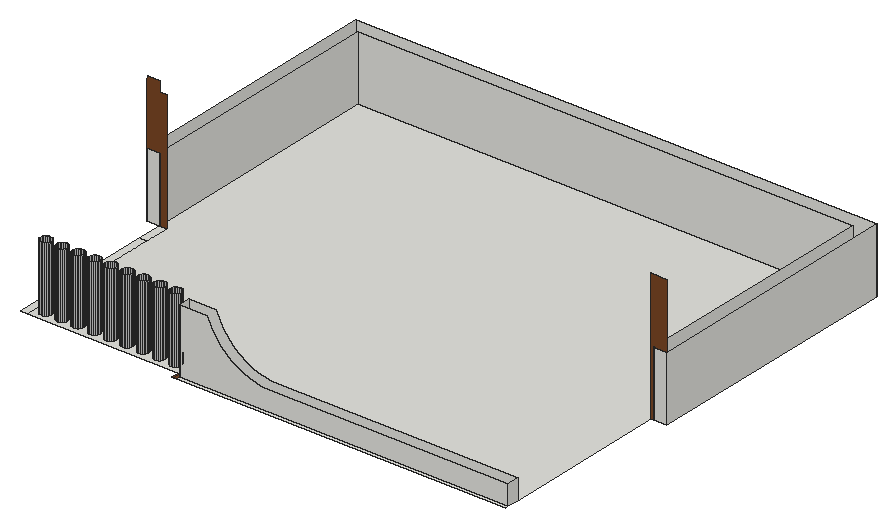
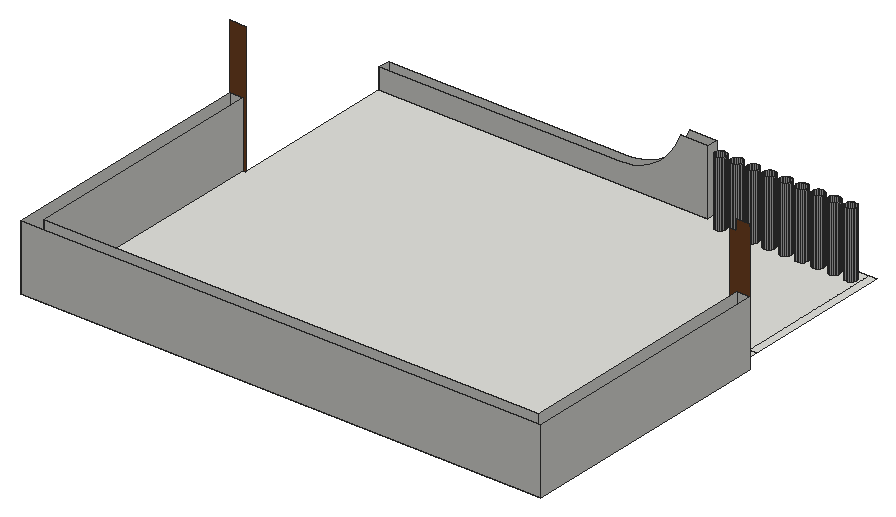
# SketchUp Ruby script. Lengths in millimetres.
U = 1.mm
M = Sketchup.active_model
def pt(a) = Geom::Point3d.new(a.map { |v| v * U })
def face(e, loops, mat)
  f = e.add_face(loops[0].map { |a| pt(a) })
  loops[1..].each { |l| e.add_face(l.map { |a| pt(a) }).erase! }
  f.material = f.back_material = mat if mat
  f
end
# faces: each face lists its corners as indices into pts; further lists are holes
def faces(e, pts, list, mat = nil) = list.each { |f| face(e, (f[0].is_a?(Array) ? f : [f]).map { |l| l.map { |i| pts[i] } }, mat) }
# xy, xz, yz: faces in a plane at the given z, y or x. An outline is a flat list of corners, or four numbers for a rectangle; further outlines are holes
def ring(l) = l.size == 4 ? [[l[0], l[1]], [l[2], l[1]], [l[2], l[3]], [l[0], l[3]]] : l.each_slice(2).to_a
def flat(e, list, mat, &to3) = list.each { |f| face(e, (f[0].is_a?(Array) ? f : [f]).map { |l| ring(l).map { |u, v| to3.(u, v) } }, mat) }
def xy(e, z, list, mat = nil) = flat(e, list, mat) { |x, y| [x, y, z] }
def xz(e, y, list, mat = nil) = flat(e, list, mat) { |x, z| [x, y, z] }
def yz(e, x, list, mat = nil) = flat(e, list, mat) { |y, z| [x, y, z] }
def lines(e, pts, list) = list.each { |a, b| e.add_line(pt(pts[a]), pt(pts[b])) }
# prism: a flat outline (further loops are holes) pulled along v
def prism(e, loops, v, mat = nil)
  f = face(e, loops, mat); d = Geom::Vector3d.new(v.map { |x| x * U })
  f.pushpull(f.normal.samedirection?(d) ? d.length : -d.length)
end
def box(e, o, s, mat = nil) = prism(e, [[o, [o[0] + s[0], o[1], o[2]], [o[0] + s[0], o[1] + s[1], o[2]], [o[0], o[1] + s[1], o[2]]]], [0, 0, s[2]], mat)
def at(x, y, z, deg = 0) = Geom::Transformation.translation(pt([x, y, z])) * Geom::Transformation.rotation(ORIGIN, Z_AXIS, deg.degrees)
def axes(o, x, y, z) = Geom::Transformation.new([*x, 0, *y, 0, *z, 0, *pt(o).to_a, 1])
def part(name) = M.definitions.add(name)
# library, detail: a bought-in or finely detailed component or shape, given as its bounding box
def library(name, o, s) = part(name).tap { |d| box(d.entities, o, s) }
def detail(e, o, s) = box(e.add_group.entities, o, s)
def put(e, d, t, mat = nil) = e.add_instance(d, t).tap { |i| i.material = mat if mat }
def group(e, t, mat = nil) = e.add_group.tap { |g| g.transformation = t; g.material = mat if mat }.entities
root = M.entities
M.materials.add("[Metal Corrugated Shiny]").color = [193, 193, 193]
M.materials.add("[Wood Veneer 01]").color = [120, 70, 37]
xy(root,7289.8,[[[4112.5,514.4,11814.3,514.4,11814.3,582.5,4124.5,582.5,4124.5,849.3,11814.3,849.3,11814.3,4760.9,11890.5,4760.9,11890.5,10572.8,308.1,10572.8,308.1,4760.9,479.5,4760.9,479.5,687.4,4112.5,687.4],[1458.7,818.4,1424.6,822.5,1392.7,835.4,1365.2,856,1344,883.1,1330.5,914.8,1325.6,948.8,1329.8,983,1342.6,1014.9,1363.3,1042.4,1390.3,1063.6,1422,1077.1,1456,1081.9,1490.2,1077.8,1522.1,1064.9,1549.6,1044.3,1570.8,1017.2,1584.3,985.6,1589.1,951.5,1585,917.4,1572.2,885.5,1551.5,858,1524.4,836.7,1492.8,823.2],[1839.7,818.4,1805.6,822.5,1773.7,835.4,1746.2,856,1725,883.1,1711.5,914.8,1706.6,948.8,1710.8,983,1723.6,1014.9,1744.3,1042.4,1771.3,1063.6,1803,1077.1,1837,1081.9,1871.2,1077.8,1903.1,1064.9,1930.6,1044.3,1951.8,1017.2,1965.3,985.6,1970.1,951.5,1966,917.4,1953.2,885.5,1932.5,858,1905.4,836.7,1873.8,823.2],[2220.7,818.4,2186.6,822.5,2154.7,835.4,2127.2,856,2106,883.1,2092.5,914.8,2087.6,948.8,2091.8,983,2104.6,1014.9,2125.3,1042.4,2152.3,1063.6,2184,1077.1,2218,1081.9,2252.2,1077.8,2284.1,1064.9,2311.6,1044.3,2332.8,1017.2,2346.3,985.6,2351.1,951.5,2347,917.4,2334.2,885.5,2313.5,858,2286.4,836.7,2254.8,823.2],[1077.7,818.4,1043.6,822.5,1011.7,835.4,984.2,856,963,883.1,949.5,914.8,944.6,948.8,948.8,983,961.6,1014.9,982.3,1042.4,1009.3,1063.6,1041,1077.1,1075,1081.9,1109.2,1077.8,1141.1,1064.9,1168.6,1044.3,1189.8,1017.2,1203.3,985.6,1208.1,951.5,1204,917.4,1191.2,885.5,1170.5,858,1143.4,836.7,1111.8,823.2],[696.7,818.4,662.6,822.5,630.7,835.4,603.2,856,582,883.1,568.5,914.8,563.6,948.8,567.8,983,580.6,1014.9,601.3,1042.4,628.3,1063.6,660,1077.1,694,1081.9,728.2,1077.8,760.1,1064.9,787.6,1044.3,808.8,1017.2,822.3,985.6,827.1,951.5,823,917.4,810.2,885.5,789.5,858,762.4,836.7,730.8,823.2],[2601.7,818.4,2567.6,822.5,2535.7,835.4,2508.2,856,2487,883.1,2473.5,914.8,2468.6,948.8,2472.8,983,2485.6,1014.9,2506.3,1042.4,2533.3,1063.6,2565,1077.1,2599,1081.9,2633.2,1077.8,2665.1,1064.9,2692.6,1044.3,2713.8,1017.2,2727.3,985.6,2732.1,951.5,2728,917.4,2715.2,885.5,2694.5,858,2667.4,836.7,2635.8,823.2],[2982.7,818.4,2948.6,822.5,2916.7,835.4,2889.2,856,2868,883.1,2854.5,914.8,2849.6,948.8,2853.8,983,2866.6,1014.9,2887.3,1042.4,2914.3,1063.6,2946,1077.1,2980,1081.9,3014.2,1077.8,3046.1,1064.9,3073.6,1044.3,3094.8,1017.2,3108.3,985.6,3113.1,951.5,3109,917.4,3096.2,885.5,3075.5,858,3048.4,836.7,3016.8,823.2],[3363.7,818.4,3329.6,822.5,3297.7,835.4,3270.2,856,3249,883.1,3235.5,914.8,3230.6,948.8,3234.8,983,3247.6,1014.9,3268.3,1042.4,3295.3,1063.6,3327,1077.1,3361,1081.9,3395.2,1077.8,3427.1,1064.9,3454.6,1044.3,3475.8,1017.2,3489.3,985.6,3494.1,951.5,3490,917.4,3477.2,885.5,3456.5,858,3429.4,836.7,3397.8,823.2],[3744.7,818.4,3710.6,822.5,3678.7,835.4,3651.2,856,3630,883.1,3616.5,914.8,3611.6,948.8,3615.8,983,3628.6,1014.9,3649.3,1042.4,3676.3,1063.6,3708,1077.1,3742,1081.9,3776.2,1077.8,3808.1,1064.9,3835.6,1044.3,3856.8,1017.2,3870.3,985.6,3875.1,951.5,3871,917.4,3858.2,885.5,3837.5,858,3810.4,836.7,3778.8,823.2]],[4124.5,582.5,11814.3,849.3],[308.1,687.4,479.5,4181.5],[308.1,4181.5,479.5,4760.9],[3.3,4760.9,3.3,10877.6,12195.3,10877.6,12195.3,4760.9,11890.5,4760.9,11890.5,10572.8,308.1,10572.8,308.1,4760.9]])
xy(root,7289.8,[[696.7,818.4,662.6,822.5,630.7,835.4,603.2,856,582,883.1,568.5,914.8,563.6,948.8,567.8,983,580.6,1014.9,601.3,1042.4,628.3,1063.6,660,1077.1,694,1081.9,728.2,1077.8,760.1,1064.9,787.6,1044.3,808.8,1017.2,822.3,985.6,827.1,951.5,823,917.4,810.2,885.5,789.5,858,762.4,836.7,730.8,823.2],[1077.7,818.4,1043.6,822.5,1011.7,835.4,984.2,856,963,883.1,949.5,914.8,944.6,948.8,948.8,983,961.6,1014.9,982.3,1042.4,1009.3,1063.6,1041,1077.1,1075,1081.9,1109.2,1077.8,1141.1,1064.9,1168.6,1044.3,1189.8,1017.2,1203.3,985.6,1208.1,951.5,1204,917.4,1191.2,885.5,1170.5,858,1143.4,836.7,1111.8,823.2],[1458.7,818.4,1424.6,822.5,1392.7,835.4,1365.2,856,1344,883.1,1330.5,914.8,1325.6,948.8,1329.8,983,1342.6,1014.9,1363.3,1042.4,1390.3,1063.6,1422,1077.1,1456,1081.9,1490.2,1077.8,1522.1,1064.9,1549.6,1044.3,1570.8,1017.2,1584.3,985.6,1589.1,951.5,1585,917.4,1572.2,885.5,1551.5,858,1524.4,836.7,1492.8,823.2],[1839.7,818.4,1805.6,822.5,1773.7,835.4,1746.2,856,1725,883.1,1711.5,914.8,1706.6,948.8,1710.8,983,1723.6,1014.9,1744.3,1042.4,1771.3,1063.6,1803,1077.1,1837,1081.9,1871.2,1077.8,1903.1,1064.9,1930.6,1044.3,1951.8,1017.2,1965.3,985.6,1970.1,951.5,1966,917.4,1953.2,885.5,1932.5,858,1905.4,836.7,1873.8,823.2],[2220.7,818.4,2186.6,822.5,2154.7,835.4,2127.2,856,2106,883.1,2092.5,914.8,2087.6,948.8,2091.8,983,2104.6,1014.9,2125.3,1042.4,2152.3,1063.6,2184,1077.1,2218,1081.9,2252.2,1077.8,2284.1,1064.9,2311.6,1044.3,2332.8,1017.2,2346.3,985.6,2351.1,951.5,2347,917.4,2334.2,885.5,2313.5,858,2286.4,836.7,2254.8,823.2],
  [2601.7,818.4,2567.6,822.5,2535.7,835.4,2508.2,856,2487,883.1,2473.5,914.8,2468.6,948.8,2472.8,983,2485.6,1014.9,2506.3,1042.4,2533.3,1063.6,2565,1077.1,2599,1081.9,2633.2,1077.8,2665.1,1064.9,2692.6,1044.3,2713.8,1017.2,2727.3,985.6,2732.1,951.5,2728,917.4,2715.2,885.5,2694.5,858,2667.4,836.7,2635.8,823.2],[2982.7,818.4,2948.6,822.5,2916.7,835.4,2889.2,856,2868,883.1,2854.5,914.8,2849.6,948.8,2853.8,983,2866.6,1014.9,2887.3,1042.4,2914.3,1063.6,2946,1077.1,2980,1081.9,3014.2,1077.8,3046.1,1064.9,3073.6,1044.3,3094.8,1017.2,3108.3,985.6,3113.1,951.5,3109,917.4,3096.2,885.5,3075.5,858,3048.4,836.7,3016.8,823.2],[3363.7,818.4,3329.6,822.5,3297.7,835.4,3270.2,856,3249,883.1,3235.5,914.8,3230.6,948.8,3234.8,983,3247.6,1014.9,3268.3,1042.4,3295.3,1063.6,3327,1077.1,3361,1081.9,3395.2,1077.8,3427.1,1064.9,3454.6,1044.3,3475.8,1017.2,3489.3,985.6,3494.1,951.5,3490,917.4,3477.2,885.5,3456.5,858,3429.4,836.7,3397.8,823.2],[3744.7,818.4,3710.6,822.5,3678.7,835.4,3651.2,856,3630,883.1,3616.5,914.8,3611.6,948.8,3615.8,983,3628.6,1014.9,3649.3,1042.4,3676.3,1063.6,3708,1077.1,3742,1081.9,3776.2,1077.8,3808.1,1064.9,3835.6,1044.3,3856.8,1017.2,3870.3,985.6,3875.1,951.5,3871,917.4,3858.2,885.5,3837.5,858,3810.4,836.7,3778.8,823.2]],"[Metal Corrugated Shiny]")
xz(root,582.5,[[4124.5,7289.8,11814.3,7289.8,11814.3,7765.4,6213.6,7765.4,6054.6,7773.7,5897.3,7798.5,5743.5,7839.6,5594.8,7896.5,5452.9,7968.5,5319.2,8055,5195.3,8154.9,5082.4,8267.2,4981.9,8390.6,4894.7,8523.8,4822,8665.4,4764.3,8813.8,4124.5,8813.8]])
xz(root,849.3,[[4124.5,7289.8,4124.5,8813.8,4764.3,8813.8,4822,8665.4,4894.7,8523.8,4981.9,8390.6,5082.4,8267.2,5195.3,8154.9,5319.2,8055,5452.9,7968.5,5594.8,7896.5,5743.5,7839.6,5897.3,7798.5,6054.6,7773.7,6213.6,7765.4,11814.3,7765.4,11814.3,7289.8]])
xz(root,4760.9,[[3.3,7289.8,308.1,8813.8],[11890.5,7289.8,12195.3,8813.8]])
xz(root,4760.9,[[308.1,7289.8,308.1,8813.8,3.3,8813.8,3.3,10221.2,7.1,10258.4,24.3,10325.9,29.4,10337.8,308.1,10337.8,308.1,10096.5,479.5,10096.5,479.5,7289.8],[11814.3,7289.8,11814.3,10337.8,12195.3,10337.8,12195.3,8813.8,11890.5,8813.8,11890.5,7289.8]],"[Wood Veneer 01]")
xz(root,10572.8,[[308.1,7289.8,11890.5,8813.8]])
xz(root,10877.6,[[3.3,7289.8,12195.3,8813.8]])
yz(root,3.3,[[4760.9,7289.8,10877.6,8813.8]])
yz(root,308.1,[[4760.9,7289.8,10572.8,8813.8]])
yz(root,4124.5,[[582.5,7289.8,849.3,8813.8]])
yz(root,11814.3,[[582.5,7289.8,849.3,7765.4]])
yz(root,11890.5,[[4760.9,7289.8,10572.8,8813.8]])
yz(root,12195.3,[[4760.9,7289.8,10877.6,8813.8]])
p = [[4048.9,687.4,7286.3],[3986.1,687.4,7276],[3986.1,514.4,7276],[4048.9,514.4,7286.3],[4112.5,687.4,7289.8],[4112.5,514.4,7289.8],
  [662.6,822.5,7289.8],[696.7,818.4,7289.8],[696.7,818.4,8813.8],[662.6,822.5,8813.8],[730.8,823.2,7289.8],[730.8,823.2,8813.8],
  [1043.6,822.5,7289.8],[1077.7,818.4,7289.8],[1077.7,818.4,8813.8],[1043.6,822.5,8813.8],[1111.8,823.2,7289.8],[1111.8,823.2,8813.8],
  [1424.6,822.5,7289.8],[1458.7,818.4,7289.8],[1458.7,818.4,8813.8],[1424.6,822.5,8813.8],[1492.8,823.2,7289.8],[1492.8,823.2,8813.8],
  [1805.6,822.5,7289.8],[1839.7,818.4,7289.8],[1839.7,818.4,8813.8],[1805.6,822.5,8813.8],[1873.8,823.2,7289.8],[1873.8,823.2,8813.8],
  [2186.6,822.5,7289.8],[2220.7,818.4,7289.8],[2220.7,818.4,8813.8],[2186.6,822.5,8813.8],[2254.8,823.2,7289.8],[2254.8,823.2,8813.8],
  [2567.6,822.5,7289.8],[2601.7,818.4,7289.8],[2601.7,818.4,8813.8],[2567.6,822.5,8813.8],[2635.8,823.2,7289.8],[2635.8,823.2,8813.8],
  [2948.6,822.5,7289.8],[2982.7,818.4,7289.8],[2982.7,818.4,8813.8],[2948.6,822.5,8813.8],[3016.8,823.2,7289.8],[3016.8,823.2,8813.8],
  [3329.6,822.5,7289.8],[3363.7,818.4,7289.8],[3363.7,818.4,8813.8],[3329.6,822.5,8813.8],[3397.8,823.2,7289.8],[3397.8,823.2,8813.8],
  [3710.6,822.5,7289.8],[3744.7,818.4,7289.8],[3744.7,818.4,8813.8],[3710.6,822.5,8813.8],[3778.8,823.2,7289.8],[3778.8,823.2,8813.8],
  [630.7,835.4,7289.8],[630.7,835.4,8813.8],[1011.7,835.4,7289.8],[1011.7,835.4,8813.8],[1392.7,835.4,7289.8],[1392.7,835.4,8813.8],
  [1773.7,835.4,7289.8],[1773.7,835.4,8813.8],[2154.7,835.4,7289.8],[2154.7,835.4,8813.8],[2535.7,835.4,7289.8],[2535.7,835.4,8813.8],
  [2916.7,835.4,7289.8],[2916.7,835.4,8813.8],[3297.7,835.4,7289.8],[3297.7,835.4,8813.8],[3678.7,835.4,7289.8],[3678.7,835.4,8813.8],
  [762.4,836.7,7289.8],[762.4,836.7,8813.8],[1143.4,836.7,7289.8],[1143.4,836.7,8813.8],[1524.4,836.7,7289.8],[1524.4,836.7,8813.8],
  [1905.4,836.7,7289.8],[1905.4,836.7,8813.8],[2286.4,836.7,7289.8],[2286.4,836.7,8813.8],[2667.4,836.7,7289.8],[2667.4,836.7,8813.8],
  [3048.4,836.7,7289.8],[3048.4,836.7,8813.8],[3429.4,836.7,7289.8],[3429.4,836.7,8813.8],[3810.4,836.7,7289.8],[3810.4,836.7,8813.8],
  [603.2,856,7289.8],[603.2,856,8813.8],[984.2,856,7289.8],[984.2,856,8813.8],[1365.2,856,7289.8],[1365.2,856,8813.8],
  [1746.2,856,7289.8],[1746.2,856,8813.8],[2127.2,856,7289.8],[2127.2,856,8813.8],[2508.2,856,7289.8],[2508.2,856,8813.8],
  [2889.2,856,7289.8],[2889.2,856,8813.8],[3270.2,856,7289.8],[3270.2,856,8813.8],[3651.2,856,7289.8],[3651.2,856,8813.8],
  [789.5,858,7289.8],[789.5,858,8813.8],[1170.5,858,7289.8],[1170.5,858,8813.8],[1551.5,858,7289.8],[1551.5,858,8813.8],
  [1932.5,858,7289.8],[1932.5,858,8813.8],[2313.5,858,7289.8],[2313.5,858,8813.8],[2694.5,858,7289.8],[2694.5,858,8813.8],
  [3075.5,858,7289.8],[3075.5,858,8813.8],[3456.5,858,7289.8],[3456.5,858,8813.8],[3837.5,858,7289.8],[3837.5,858,8813.8],
  [582,883.1,7289.8],[582,883.1,8813.8],[963,883.1,7289.8],[963,883.1,8813.8],[1344,883.1,7289.8],[1344,883.1,8813.8],
  [1725,883.1,7289.8],[1725,883.1,8813.8],[2106,883.1,7289.8],[2106,883.1,8813.8],[2487,883.1,7289.8],[2487,883.1,8813.8],
  [2868,883.1,7289.8],[2868,883.1,8813.8],[3249,883.1,7289.8],[3249,883.1,8813.8],[3630,883.1,7289.8],[3630,883.1,8813.8],
  [810.2,885.5,7289.8],[810.2,885.5,8813.8],[1191.2,885.5,7289.8],[1191.2,885.5,8813.8],[1572.2,885.5,7289.8],[1572.2,885.5,8813.8],
  [1953.2,885.5,7289.8],[1953.2,885.5,8813.8],[2334.2,885.5,7289.8],[2334.2,885.5,8813.8],[2715.2,885.5,7289.8],[2715.2,885.5,8813.8],
  [3096.2,885.5,7289.8],[3096.2,885.5,8813.8],[3477.2,885.5,7289.8],[3477.2,885.5,8813.8],[3858.2,885.5,7289.8],[3858.2,885.5,8813.8],
  [568.5,914.8,7289.8],[568.5,914.8,8813.8],[949.5,914.8,7289.8],[949.5,914.8,8813.8],[1330.5,914.8,7289.8],[1330.5,914.8,8813.8],
  [1711.5,914.8,7289.8],[1711.5,914.8,8813.8],[2092.5,914.8,7289.8],[2092.5,914.8,8813.8],[2473.5,914.8,7289.8],[2473.5,914.8,8813.8],
  [2854.5,914.8,7289.8],[2854.5,914.8,8813.8],[3235.5,914.8,7289.8],[3235.5,914.8,8813.8],[3616.5,914.8,7289.8],[3616.5,914.8,8813.8],
  [823,917.4,7289.8],[823,917.4,8813.8],[1204,917.4,7289.8],[1204,917.4,8813.8],[1585,917.4,7289.8],[1585,917.4,8813.8],
  [1966,917.4,7289.8],[1966,917.4,8813.8],[2347,917.4,7289.8],[2347,917.4,8813.8],[2728,917.4,7289.8],[2728,917.4,8813.8],
  [3109,917.4,7289.8],[3109,917.4,8813.8],[3490,917.4,7289.8],[3490,917.4,8813.8],[3871,917.4,7289.8],[3871,917.4,8813.8],
  [563.6,948.8,7289.8],[563.6,948.8,8813.8],[944.6,948.8,7289.8],[944.6,948.8,8813.8],[1325.6,948.8,7289.8],[1325.6,948.8,8813.8],
  [1706.6,948.8,7289.8],[1706.6,948.8,8813.8],[2087.6,948.8,7289.8],[2087.6,948.8,8813.8],[2468.6,948.8,7289.8],[2468.6,948.8,8813.8],
  [2849.6,948.8,7289.8],[2849.6,948.8,8813.8],[3230.6,948.8,7289.8],[3230.6,948.8,8813.8],[3611.6,948.8,7289.8],[3611.6,948.8,8813.8],
  [827.1,951.5,7289.8],[827.1,951.5,8813.8],[1208.1,951.5,7289.8],[1208.1,951.5,8813.8],[1589.1,951.5,7289.8],[1589.1,951.5,8813.8],
  [1970.1,951.5,7289.8],[1970.1,951.5,8813.8],[2351.1,951.5,7289.8],[2351.1,951.5,8813.8],[2732.1,951.5,7289.8],[2732.1,951.5,8813.8],
  [3113.1,951.5,7289.8],[3113.1,951.5,8813.8],[3494.1,951.5,7289.8],[3494.1,951.5,8813.8],[3875.1,951.5,7289.8],[3875.1,951.5,8813.8],
  [567.8,983,7289.8],[567.8,983,8813.8],[948.8,983,7289.8],[948.8,983,8813.8],[1329.8,983,7289.8],[1329.8,983,8813.8],
  [1710.8,983,7289.8],[1710.8,983,8813.8],[2091.8,983,7289.8],[2091.8,983,8813.8],[2472.8,983,7289.8],[2472.8,983,8813.8],
  [2853.8,983,7289.8],[2853.8,983,8813.8],[3234.8,983,7289.8],[3234.8,983,8813.8],[3615.8,983,7289.8],[3615.8,983,8813.8],
  [822.3,985.6,7289.8],[822.3,985.6,8813.8],[1203.3,985.6,7289.8],[1203.3,985.6,8813.8],[1584.3,985.6,7289.8],[1584.3,985.6,8813.8],
  [1965.3,985.6,7289.8],[1965.3,985.6,8813.8],[2346.3,985.6,7289.8],[2346.3,985.6,8813.8],[2727.3,985.6,7289.8],[2727.3,985.6,8813.8],
  [3108.3,985.6,7289.8],[3108.3,985.6,8813.8],[3489.3,985.6,7289.8],[3489.3,985.6,8813.8],[3870.3,985.6,7289.8],[3870.3,985.6,8813.8],
  [580.6,1014.9,7289.8],[580.6,1014.9,8813.8],[961.6,1014.9,7289.8],[961.6,1014.9,8813.8],[1342.6,1014.9,7289.8],[1342.6,1014.9,8813.8],
  [1723.6,1014.9,7289.8],[1723.6,1014.9,8813.8],[2104.6,1014.9,7289.8],[2104.6,1014.9,8813.8],[2485.6,1014.9,7289.8],[2485.6,1014.9,8813.8],
  [2866.6,1014.9,7289.8],[2866.6,1014.9,8813.8],[3247.6,1014.9,7289.8],[3247.6,1014.9,8813.8],[3628.6,1014.9,7289.8],[3628.6,1014.9,8813.8],
  [808.8,1017.2,7289.8],[808.8,1017.2,8813.8],[1189.8,1017.2,7289.8],[1189.8,1017.2,8813.8],[1570.8,1017.2,7289.8],[1570.8,1017.2,8813.8],
  [1951.8,1017.2,7289.8],[1951.8,1017.2,8813.8],[2332.8,1017.2,7289.8],[2332.8,1017.2,8813.8],[2713.8,1017.2,7289.8],[2713.8,1017.2,8813.8],
  [3094.8,1017.2,7289.8],[3094.8,1017.2,8813.8],[3475.8,1017.2,7289.8],[3475.8,1017.2,8813.8],[3856.8,1017.2,7289.8],[3856.8,1017.2,8813.8],
  [601.3,1042.4,7289.8],[601.3,1042.4,8813.8],[982.3,1042.4,7289.8],[982.3,1042.4,8813.8],[1363.3,1042.4,7289.8],[1363.3,1042.4,8813.8],
  [1744.3,1042.4,7289.8],[1744.3,1042.4,8813.8],[2125.3,1042.4,7289.8],[2125.3,1042.4,8813.8],[2506.3,1042.4,7289.8],[2506.3,1042.4,8813.8],
  [2887.3,1042.4,7289.8],[2887.3,1042.4,8813.8],[3268.3,1042.4,7289.8],[3268.3,1042.4,8813.8],[3649.3,1042.4,7289.8],[3649.3,1042.4,8813.8],
  [787.6,1044.3,7289.8],[787.6,1044.3,8813.8],[1168.6,1044.3,7289.8],[1168.6,1044.3,8813.8],[1549.6,1044.3,7289.8],[1549.6,1044.3,8813.8],
  [1930.6,1044.3,7289.8],[1930.6,1044.3,8813.8],[2311.6,1044.3,7289.8],[2311.6,1044.3,8813.8],[2692.6,1044.3,7289.8],[2692.6,1044.3,8813.8],
  [3073.6,1044.3,7289.8],[3073.6,1044.3,8813.8],[3454.6,1044.3,7289.8],[3454.6,1044.3,8813.8],[3835.6,1044.3,7289.8],[3835.6,1044.3,8813.8],
  [628.3,1063.6,7289.8],[628.3,1063.6,8813.8],[1009.3,1063.6,7289.8],[1009.3,1063.6,8813.8],[1390.3,1063.6,7289.8],[1390.3,1063.6,8813.8],
  [1771.3,1063.6,7289.8],[1771.3,1063.6,8813.8],[2152.3,1063.6,7289.8],[2152.3,1063.6,8813.8],[2533.3,1063.6,7289.8],[2533.3,1063.6,8813.8],
  [2914.3,1063.6,7289.8],[2914.3,1063.6,8813.8],[3295.3,1063.6,7289.8],[3295.3,1063.6,8813.8],[3676.3,1063.6,7289.8],[3676.3,1063.6,8813.8],
  [760.1,1064.9,7289.8],[760.1,1064.9,8813.8],[1141.1,1064.9,7289.8],[1141.1,1064.9,8813.8],[1522.1,1064.9,7289.8],[1522.1,1064.9,8813.8],
  [1903.1,1064.9,7289.8],[1903.1,1064.9,8813.8],[2284.1,1064.9,7289.8],[2284.1,1064.9,8813.8],[2665.1,1064.9,7289.8],[2665.1,1064.9,8813.8],
  [3046.1,1064.9,7289.8],[3046.1,1064.9,8813.8],[3427.1,1064.9,7289.8],[3427.1,1064.9,8813.8],[3808.1,1064.9,7289.8],[3808.1,1064.9,8813.8],
  [660,1077.1,7289.8],[660,1077.1,8813.8],[1041,1077.1,7289.8],[1041,1077.1,8813.8],[1422,1077.1,7289.8],[1422,1077.1,8813.8],
  [1803,1077.1,7289.8],[1803,1077.1,8813.8],[2184,1077.1,7289.8],[2184,1077.1,8813.8],[2565,1077.1,7289.8],[2565,1077.1,8813.8],
  [2946,1077.1,7289.8],[2946,1077.1,8813.8],[3327,1077.1,7289.8],[3327,1077.1,8813.8],[3708,1077.1,7289.8],[3708,1077.1,8813.8],
  [728.2,1077.8,7289.8],[728.2,1077.8,8813.8],[1109.2,1077.8,7289.8],[1109.2,1077.8,8813.8],[1490.2,1077.8,7289.8],[1490.2,1077.8,8813.8],
  [1871.2,1077.8,7289.8],[1871.2,1077.8,8813.8],[2252.2,1077.8,7289.8],[2252.2,1077.8,8813.8],[2633.2,1077.8,7289.8],[2633.2,1077.8,8813.8],
  [3014.2,1077.8,7289.8],[3014.2,1077.8,8813.8],[3395.2,1077.8,7289.8],[3395.2,1077.8,8813.8],[3776.2,1077.8,7289.8],[3776.2,1077.8,8813.8],
  [694,1081.9,7289.8],[694,1081.9,8813.8],[1075,1081.9,7289.8],[1075,1081.9,8813.8],[1456,1081.9,7289.8],[1456,1081.9,8813.8],
  [1837,1081.9,7289.8],[1837,1081.9,8813.8],[2218,1081.9,7289.8],[2218,1081.9,8813.8],[2599,1081.9,7289.8],[2599,1081.9,8813.8],
  [2980,1081.9,7289.8],[2980,1081.9,8813.8],[3361,1081.9,7289.8],[3361,1081.9,8813.8],[3742,1081.9,7289.8],[3742,1081.9,8813.8]]
faces(root,p,[[0,1,2,3],[4,0,3,5]],"[Wood Veneer 01]")
faces(root,p,[[6,7,8,9],[7,10,11,8],[12,13,14,15],[13,16,17,14],[18,19,20,21],[19,22,23,20],[24,25,26,27],[25,28,29,26],
  [30,31,32,33],[31,34,35,32],[36,37,38,39],[37,40,41,38],[42,43,44,45],[43,46,47,44],[48,49,50,51],[49,52,53,50],
  [54,55,56,57],[55,58,59,56],[60,6,9,61],[62,12,15,63],[64,18,21,65],[66,24,27,67],[68,30,33,69],[70,36,39,71],
  [72,42,45,73],[74,48,51,75],[76,54,57,77],[10,78,79,11],[16,80,81,17],[22,82,83,23],[28,84,85,29],[34,86,87,35],
  [40,88,89,41],[46,90,91,47],[52,92,93,53],[58,94,95,59],[96,60,61,97],[98,62,63,99],[100,64,65,101],[102,66,67,103],
  [104,68,69,105],[106,70,71,107],[108,72,73,109],[110,74,75,111],[112,76,77,113],[78,114,115,79],[80,116,117,81],[82,118,119,83],
  [84,120,121,85],[86,122,123,87],[88,124,125,89],[90,126,127,91],[92,128,129,93],[94,130,131,95],[132,96,97,133],[134,98,99,135],
  [136,100,101,137],[138,102,103,139],[140,104,105,141],[142,106,107,143],[144,108,109,145],[146,110,111,147],[148,112,113,149],[114,150,151,115],
  [116,152,153,117],[118,154,155,119],[120,156,157,121],[122,158,159,123],[124,160,161,125],[126,162,163,127],[128,164,165,129],[130,166,167,131],
  [168,132,133,169],[170,134,135,171],[172,136,137,173],[174,138,139,175],[176,140,141,177],[178,142,143,179],[180,144,145,181],[182,146,147,183],
  [184,148,149,185],[150,186,187,151],[152,188,189,153],[154,190,191,155],[156,192,193,157],[158,194,195,159],[160,196,197,161],[162,198,199,163],
  [164,200,201,165],[166,202,203,167],[204,168,169,205],[206,170,171,207],[208,172,173,209],[210,174,175,211],[212,176,177,213],[214,178,179,215],
  [216,180,181,217],[218,182,183,219],[220,184,185,221],[186,222,223,187],[188,224,225,189],[190,226,227,191],[192,228,229,193],[194,230,231,195],
  [196,232,233,197],[198,234,235,199],[200,236,237,201],[202,238,239,203],[240,204,205,241],[242,206,207,243],[244,208,209,245],[246,210,211,247],
  [248,212,213,249],[250,214,215,251],[252,216,217,253],[254,218,219,255],[256,220,221,257],[222,258,259,223],[224,260,261,225],[226,262,263,227],
  [228,264,265,229],[230,266,267,231],[232,268,269,233],[234,270,271,235],[236,272,273,237],[238,274,275,239],[276,240,241,277],[278,242,243,279],
  [280,244,245,281],[282,246,247,283],[284,248,249,285],[286,250,251,287],[288,252,253,289],[290,254,255,291],[292,256,257,293],[258,294,295,259],
  [260,296,297,261],[262,298,299,263],[264,300,301,265],[266,302,303,267],[268,304,305,269],[270,306,307,271],[272,308,309,273],[274,310,311,275],
  [312,276,277,313],[314,278,279,315],[316,280,281,317],[318,282,283,319],[320,284,285,321],[322,286,287,323],[324,288,289,325],[326,290,291,327],
  [328,292,293,329],[294,330,331,295],[296,332,333,297],[298,334,335,299],[300,336,337,301],[302,338,339,303],[304,340,341,305],[306,342,343,307],
  [308,344,345,309],[310,346,347,311],[348,312,313,349],[350,314,315,351],[352,316,317,353],[354,318,319,355],[356,320,321,357],[358,322,323,359],
  [360,324,325,361],[362,326,327,363],[364,328,329,365],[330,366,367,331],[332,368,369,333],[334,370,371,335],[336,372,373,337],[338,374,375,339],
  [340,376,377,341],[342,378,379,343],[344,380,381,345],[346,382,383,347],[384,348,349,385],[386,350,351,387],[388,352,353,389],[390,354,355,391],
  [392,356,357,393],[394,358,359,395],[396,360,361,397],[398,362,363,399],[400,364,365,401],[366,402,403,367],[368,404,405,369],[370,406,407,371],
  [372,408,409,373],[374,410,411,375],[376,412,413,377],[378,414,415,379],[380,416,417,381],[382,418,419,383],[420,384,385,421],[422,386,387,423],
  [424,388,389,425],[426,390,391,427],[428,392,393,429],[430,394,395,431],[432,396,397,433],[434,398,399,435],[436,400,401,437],[402,420,421,403],
  [404,422,423,405],[406,424,425,407],[408,426,427,409],[410,428,429,411],[412,430,431,413],[414,432,433,415],[416,434,435,417],[418,436,437,419]],"[Metal Corrugated Shiny]")
